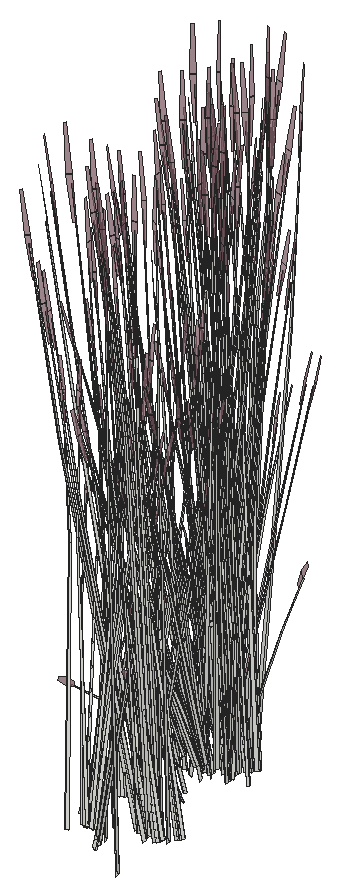
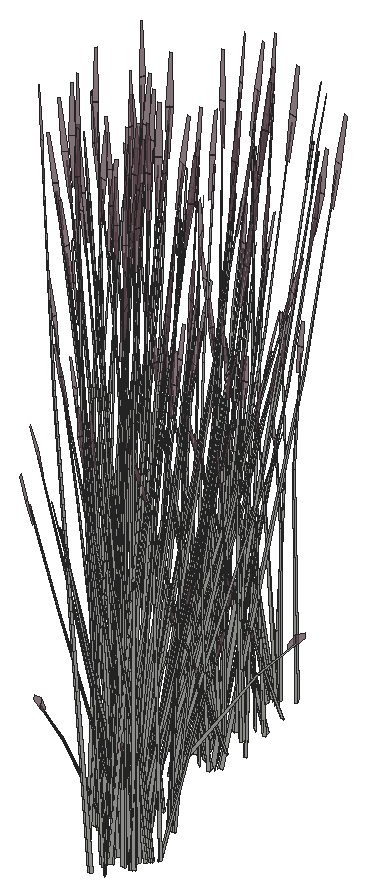
# SketchUp Ruby script. Lengths in inches.
U = 1.inch
M = Sketchup.active_model
def pt(a) = Geom::Point3d.new(a.map { |v| v * U })
def face(e, loops, mat)
  f = e.add_face(loops[0].map { |a| pt(a) })
  loops[1..].each { |l| e.add_face(l.map { |a| pt(a) }).erase! }
  f.material = f.back_material = mat if mat
  f
end
# faces: each face lists its corners as indices into pts; further lists are holes
def faces(e, pts, list, mat = nil) = list.each { |f| face(e, (f[0].is_a?(Array) ? f : [f]).map { |l| l.map { |i| pts[i] } }, mat) }
# xy, xz, yz: faces in a plane at the given z, y or x. An outline is a flat list of corners, or four numbers for a rectangle; further outlines are holes
def ring(l) = l.size == 4 ? [[l[0], l[1]], [l[2], l[1]], [l[2], l[3]], [l[0], l[3]]] : l.each_slice(2).to_a
def flat(e, list, mat, &to3) = list.each { |f| face(e, (f[0].is_a?(Array) ? f : [f]).map { |l| ring(l).map { |u, v| to3.(u, v) } }, mat) }
def xy(e, z, list, mat = nil) = flat(e, list, mat) { |x, y| [x, y, z] }
def xz(e, y, list, mat = nil) = flat(e, list, mat) { |x, z| [x, y, z] }
def yz(e, x, list, mat = nil) = flat(e, list, mat) { |y, z| [x, y, z] }
def lines(e, pts, list) = list.each { |a, b| e.add_line(pt(pts[a]), pt(pts[b])) }
# prism: a flat outline (further loops are holes) pulled along v
def prism(e, loops, v, mat = nil)
  f = face(e, loops, mat); d = Geom::Vector3d.new(v.map { |x| x * U })
  f.pushpull(f.normal.samedirection?(d) ? d.length : -d.length)
end
def box(e, o, s, mat = nil) = prism(e, [[o, [o[0] + s[0], o[1], o[2]], [o[0] + s[0], o[1] + s[1], o[2]], [o[0], o[1] + s[1], o[2]]]], [0, 0, s[2]], mat)
def at(x, y, z, deg = 0) = Geom::Transformation.translation(pt([x, y, z])) * Geom::Transformation.rotation(ORIGIN, Z_AXIS, deg.degrees)
def axes(o, x, y, z) = Geom::Transformation.new([*x, 0, *y, 0, *z, 0, *pt(o).to_a, 1])
def part(name) = M.definitions.add(name)
# library, detail: a bought-in or finely detailed component or shape, given as its bounding box
def library(name, o, s) = part(name).tap { |d| box(d.entities, o, s) }
def detail(e, o, s) = box(e.add_group.entities, o, s)
def put(e, d, t, mat = nil) = e.add_instance(d, t).tap { |i| i.material = mat if mat }
def group(e, t, mat = nil) = e.add_group.tap { |g| g.transformation = t; g.material = mat if mat }.entities
root = M.entities
M.materials.add("LightPink_Translucent").color = [144, 107, 117]
M.materials["LightPink_Translucent"].alpha = 0.75
c1 = part("blade")
p = [[2.15,0.21,22],[0,0.17,0],[0.09,0.45,0],[2.18,0.31,22],[2.29,0.31,22],[0.38,0.45,0],
  [2.48,0.24,33],[2.49,0.24,33],[2.48,0.22,33]]
faces(c1.entities,p,[[0,1,2,3],[4,5,2,3],[6,3,4,7],[8,0,3,6]])
c2 = part("seeds")
p = [[0.3,-0.1,1.38],[-0.01,-0.03,1.59],[-0.01,-0.03,0.03],[0.14,-0.07,-0.07],[0.29,-0.03,3],[0.15,0.01,3.11]]
faces(c2.entities,p,[[0,1,2,3],[1,0,4,5]],"LightPink_Translucent")
c3 = part("blade with seeds")
put(c3.entities,c1,at(0,0,0))
put(c3.entities,c2,axes([2.4,0.25,30.99],[1.5799,-0.05474,1.17369],[-0.12525,1.92788,0.29478],[-0.07173,-0.02425,1.56792]))
put(root,c3,axes([290.63,462.82,5.03],[0.82753,0.35977,-0.1216],[-0.47675,0.52101,-0.67495],[-0.2338,0.18111,1.02557]))
put(root,c3,axes([291.23,468.59,2.48],[0,0.65246,0.49651],[-1.00089,0,0],[0,-0.1486,1.57504]))
put(root,c3,axes([293.6,469.11,2.21],[-0.53742,-0.54764,-0.44739],[0.81403,-0.38564,0.21531],[-0.17391,-0.06776,1.43643]))
put(root,c3,axes([292.09,463.93,5.05],[0.60531,-0.34352,0.35414],[0.573,0.39225,-0.4572],[-0.08718,0.19929,0.87481]))
put(root,c3,axes([293.51,468.92,2.72],[-0.43405,0.58792,0.44739],[-0.90188,-0.28295,-0.21531],[0,-0.13553,1.43643]))
put(root,c3,axes([296.14,462.04,2.84],[-0.02444,-0.61432,1.41272],[1.10603,0.15924,0.59816],[-0.26159,0.33615,1.3335]))
put(root,c3,axes([291.54,464.24,4.73],[-0.73517,-0.0304,0.0643],[0.02016,-0.45906,0.50621],[-0.07693,0.17585,0.77189]))
put(root,c3,axes([291.77,464.28,4.73],[-0.63704,-0.44518,0.48003],[0.67652,-0.38394,0.3958],[-0.11751,0.20886,0.9933]))
put(root,c3,axes([293.8,469.06,2.36],[1.13071,0.13747,0.45755],[-0.23011,0.77639,0.17955],[-0.16524,-0.07497,1.58856]))
put(root,c3,axes([292.125,470.33,2.03],[-0.21015,-0.56852,-0.30978],[0.83462,-0.16144,0.30978],[-0.16826,-0.06556,1.38974]))
put(root,c3,axes([291.77,464.42,4.53],[-0.60531,0.34352,-0.35414],[-0.573,-0.39225,0.4572],[-0.08718,0.19929,0.87481]))
put(root,c3,axes([291.7,464.02,5.4],[0.98321,0.03233,-0.13498],[-0.02687,0.61208,-0.74919],[-0.0683,0.23574,1.13838]))
put(root,c3,axes([293.2,470.3,2.47],[0.96132,-0.17317,0.17642],[0.23737,0.64447,0.35086],[-0.08574,-0.0939,1.60407]))
put(root,c3,axes([292.15,465.75,2.77],[-0.02315,-0.38796,1.1486],[0.57853,0.27671,0.84392],[-0.11378,0.18492,0.25299]))
put(root,c3,axes([291.89,470.57,2.02],[-0.83726,-0.32623,-0.49651],[0.50045,-0.58498,0],[-0.19069,-0.0743,1.57504]))
put(root,c3,axes([294.17,469.42,2.67],[-0.90324,0.43318,-0.29095],[-0.60064,-0.61207,-0.50002],[-0.22285,-0.06216,1.59708]))
put(root,c3,axes([292.37,464.25,5],[0.64041,0.4384,-0.5672],[-0.67652,0.38394,-0.43934],[-0.09744,0.22274,1.08528]))
put(root,c3,axes([291.68,464.91,2.82],[0.8127,-0.11554,0.06507],[0.18684,0.46549,-0.86304],[-0.05152,0.23564,0.7736]))
put(root,c3,axes([294.08,469.61,2.62],[-0.17258,0.58229,0.1448],[-0.84319,-0.10108,-0.41347],[-0.15345,-0.05979,1.26744]))
put(root,c3,axes([292.17,464.05,5.34],[-0.02328,0.60353,-0.7886],[-0.98022,-0.04053,0.09517],[-0.10344,0.25568,1.11556]))
put(root,c3,axes([289.61,465.64,4.71],[0.10149,-0.03939,1.77383],[0.83886,0.26202,-0.16761],[-0.01971,0.21816,0.31391]))
put(root,c3,axes([293.1,463.625,3.875],[-0.0219,-0.25042,1.71376],[0.94901,0.16613,0.13857],[-0.0587,0.35688,0.73262]))
put(root,c3,axes([294.43,470.4,2.2],[-0.90188,-0.29293,0],[0.43405,-0.60866,0],[0,0,1.62707]))
put(root,c3,axes([295.18,469.62,2.46],[-0.87356,-0.52515,-0.25192],[0.73507,-0.5897,0.5513],[-0.23523,0.06143,1.68216]))
put(root,c3,axes([292.88,470.625,2.48],[0.83726,0.32623,0.49651],[-0.50045,0.58498,0],[-0.19069,-0.0743,1.57504]))
put(root,c3,axes([291.48,465.41,2.59],[0.28231,-0.10293,1.43002],[0.69701,0.31035,-0.30754],[-0.20746,0.26854,0.61141]))
put(root,c3,axes([292.4,470.97,2.375],[-0.55932,0.6538,0],[-0.93577,-0.36461,-0.51607],[-0.21313,-0.08304,1.63711]))
put(root,c3,axes([294.74,469.51,2.21],[-0.97146,0.04028,-0.44739],[-0.08785,-0.66859,0.21531],[-0.17391,0.06776,1.43643]))
put(root,c3,axes([291.84,464.9,3.36],[0.01966,-0.33682,1.54345],[0.88405,0.17791,0.21329],[-0.0766,0.35897,0.72882]))
put(root,c3,axes([295.82,471.06,2.19],[-0.55235,-0.65609,-0.05142],[0.93577,-0.36461,0.51607],[-0.23059,0.06247,1.6363]))
put(root,c3,axes([295.5625,470.98,2.03],[-0.83462,-0.16144,-0.30978],[0.21015,-0.56852,0.30978],[-0.16826,0.06556,1.38974]))
put(root,c3,axes([290.94,469.375,5.05],[0.77872,-0.09325,0.35414],[0.20563,0.53305,-0.4572],[-0.22316,0.14318,0.87481]))
put(root,c3,axes([295.42,469.33,2.67],[0.10425,0.7445,-0.29095],[-1.08575,0.04502,-0.50002],[-0.19119,0.09917,1.59708]))
put(root,c3,axes([291.4375,476.32,4.72],[-0.13683,-0.09148,1.74944],[-0.91315,0.058,-0.27667],[-0.14574,-0.2188,0.14031]))
put(root,c3,axes([292.4,477.86,4.98],[-0.42698,-0.53052,-0.71045],[0.87893,-0.29566,0.08574],[-0.09984,-0.25633,1.00501]))
put(root,c3,axes([291.66,476.6875,1.49],[-0.15005,0.02351,1.76342],[-0.82981,-0.26461,-0.26939],[0.01392,-0.22072,0.30037]))
put(root,c3,axes([289.17,470.89,5.65],[0.78943,0.17416,-0.06488],[-0.24284,0.53604,-0.29416],[-0.12912,0.08139,0.97024]))
put(root,c3,axes([294.77,469.9,2.06],[-0.60257,0.49041,-0.62353],[-0.74854,-0.44469,-0.16365],[-0.24146,0.12234,1.37633]))
put(root,c3,axes([295.76,471.23,2.02],[-0.83726,0.32623,-0.49651],[-0.50045,-0.58498,0],[-0.19069,0.0743,1.57504]))
put(root,c3,axes([292.48,477.41,4.53],[0.2697,-0.50175,-0.35414],[0.78684,0.14635,0.4572],[-0.07215,-0.20201,0.87481]))
put(root,c3,axes([290.53,469.33,5.03],[0.82753,0.35977,-0.1216],[-0.47675,0.52101,-0.67495],[-0.2338,0.18111,1.02557]))
put(root,c3,axes([292.07,477.76,4.68],[-0.87941,-0.16356,-0.51099],[0.30143,-0.56078,-0.3958],[-0.08064,-0.22578,0.97773]))
put(root,c3,axes([291.99,470.4375,5.05],[0.60531,-0.34352,0.35414],[0.573,0.39225,-0.4572],[-0.08718,0.19929,0.87481]))
put(root,c3,axes([296.04,468.54,2.84],[-0.02444,-0.61432,1.41272],[1.10603,0.15924,0.59816],[-0.26159,0.33615,1.3335]))
put(root,c3,axes([290.32,477.41,5.09],[0.99656,-0.1677,0.53763],[0.17295,0.65785,0.4433],[-0.23438,-0.19388,1.11249]))
put(root,c3,axes([291.4375,470.75,4.73],[-0.73517,-0.0304,0.0643],[0.02016,-0.45906,0.50621],[-0.07693,0.17585,0.77189]))
put(root,c3,axes([291.67,470.79,4.73],[-0.63704,-0.44518,0.48003],[0.67652,-0.38394,0.3958],[-0.11751,0.20886,0.9933]))
put(root,c3,axes([292.57,477.53,4.73],[0.88151,0.17057,0.48003],[-0.30143,0.56078,0.3958],[-0.05297,-0.22053,0.9933]))
put(root,c3,axes([292.83,477.73,5.03],[-0.87543,0.30377,-0.1216],[-0.4302,-0.53915,-0.67495],[-0.1155,-0.2272,1.02557]))
put(root,c3,axes([292.81,477.49,4.73],[0.6592,-0.22175,0.0643],[0.32265,0.40436,0.50621],[-0.06366,-0.17825,0.77189]))
put(root,c3,axes([290.55,477.55,4.73],[0.4066,-0.41448,0.0643],[0.57901,0.24131,0.50621],[-0.18719,-0.13288,0.77189]))
put(root,c3,axes([290.42,479.86,2.1],[-0.36739,-0.66907,-0.69835],[1.05831,-0.24096,-0.18329],[-0.04061,-0.22656,1.54149]))
put(root,c3,axes([291.67,470.92,4.53],[-0.60531,0.34352,-0.35414],[-0.573,-0.39225,0.4572],[-0.08718,0.19929,0.87481]))
put(root,c3,axes([291.6,470.53,5.4],[0.98321,0.03233,-0.13498],[-0.02687,0.61208,-0.74919],[-0.0683,0.23574,1.13838]))
put(root,c3,axes([292.5625,477.94,5.05],[-0.2697,0.50175,0.35414],[-0.78684,-0.14635,-0.4572],[-0.07215,-0.20201,0.87481]))
put(root,c3,axes([292.06,472.26,2.77],[-0.02315,-0.38796,1.1486],[0.57853,0.27671,0.84392],[-0.11378,0.18492,0.25299]))
put(root,c3,axes([291.5,477.15,2.13],[-0.61821,0.37431,-0.03893],[-0.56645,-0.40995,-0.17649],[-0.03988,-0.11616,0.58215]))
put(root,c3,axes([292.27,470.76,5],[0.64041,0.4384,-0.5672],[-0.67652,0.38394,-0.43934],[-0.09744,0.22274,1.08528]))
put(root,c3,axes([291.58,471.42,2.82],[0.8127,-0.11554,0.06507],[0.18684,0.46549,-0.86304],[-0.05152,0.23564,0.7736]))
put(root,c3,axes([292.07,470.5625,5.34],[-0.02328,0.60353,-0.7886],[-0.98022,-0.04053,0.09517],[-0.10344,0.25568,1.11556]))
put(root,c3,axes([289.51,472.15,4.71],[0.10149,-0.03939,1.77383],[0.83886,0.26202,-0.16761],[-0.01971,0.21816,0.31391]))
put(root,c3,axes([288.25,479.76,2.02],[0,-0.65246,-0.49651],[1.00089,0,0],[0,-0.1486,1.57504]))
put(root,c3,axes([293,470.13,3.875],[-0.0219,-0.25042,1.71376],[0.94901,0.16613,0.13857],[-0.0587,0.35688,0.73262]))
put(root,c3,axes([291.38,471.91,2.59],[0.28231,-0.10293,1.43002],[0.69701,0.31035,-0.30754],[-0.20746,0.26854,0.61141]))
put(root,c3,axes([290.98,480.03,2.21],[0.43405,-0.58792,-0.44739],[0.90188,0.28295,0.21531],[0,-0.13553,1.43643]))
put(root,c3,axes([288.68,479.78,2.03],[0.62448,-0.40708,-0.30978],[0.62448,0.40708,0.30978],[0,-0.13112,1.38974]))
put(root,c3,axes([290.87,480.52,2.67],[-1.00749,-0.31132,-0.29095],[0.48511,-0.65709,-0.50002],[-0.03166,-0.16133,1.59708]))
put(root,c3,axes([291.75,471.41,3.36],[0.01966,-0.33682,1.54345],[0.88405,0.17791,0.21329],[-0.0766,0.35897,0.72882]))
put(root,c3,axes([291.52,480.32,2.43],[1.00799,0.31623,0.24065],[-0.48511,0.65709,0.50002],[0,-0.15147,1.60543]))
put(root,c3,axes([291.125,481.21,2.4375],[0.23711,-0.77313,-0.23429],[1.12425,0.13477,0.51271],[-0.19645,-0.10677,1.5644]))
put(root,c3,axes([291.19,479.88,2.72],[-0.97146,0.04028,0.44739],[-0.08785,-0.66859,-0.21531],[0.17391,-0.06776,1.43643]))
put(root,c3,axes([289.57,483.67,2.59],[-0.25429,0.13207,1.43002],[-0.76157,-0.23115,-0.30754],[0.14117,-0.28747,0.61141]))
put(root,c3,axes([288.68,480.37,2.48],[0,0.65246,0.49651],[-1.00089,0,0],[0,-0.1486,1.57504]))
put(root,c3,axes([291.05,480.9,2.21],[-0.53742,-0.54764,-0.44739],[0.81403,-0.38564,0.21531],[-0.17391,-0.06776,1.43643]))
put(root,c3,axes([291.16,480.12,2.36],[0.38895,0.72959,0.45755],[-1.11135,0.2537,0.17955],[0.01358,-0.13406,1.58856]))
put(root,c3,axes([287.67,482.95,1.49],[-0.15005,0.02351,1.76342],[-0.82981,-0.26461,-0.26939],[0.01392,-0.22072,0.30037]))
put(root,c3,axes([290.96,480.7,2.72],[-0.43405,0.58792,0.44739],[-0.90188,-0.28295,-0.21531],[0,-0.13553,1.43643]))
put(root,c3,axes([292.56,480.18,2.21],[0,-0.75495,0],[1.11865,0,0],[0,0,1.79456]))
put(root,c3,axes([290.1875,484.64,4.98],[0.02328,-0.60353,-0.71045],[0.98022,0.04053,0.08574],[0.10344,-0.25568,1.00501]))
put(root,c3,axes([288.49,483.67,4.53],[0.2697,-0.50175,-0.35414],[0.78684,0.14635,0.4572],[-0.07215,-0.20201,0.87481]))
put(root,c3,axes([291.36,483.23,4.71],[-0.09085,0.04984,1.77383],[-0.89014,-0.16814,-0.16761],[-0.03222,-0.21748,0.31391]))
put(root,c3,axes([292.84,480.77,2.3],[-0.83213,-0.56158,-0.06131],[0.83263,-0.56193,0],[-0.02906,-0.01961,1.75571]))
put(root,c3,axes([290.74,478.73,2.47],[-0.25843,0.64844,0.17642],[-0.9457,-0.1835,0.35086],[0.16336,-0.00316,1.60407]))
put(root,c3,axes([288.63,482.61,2.77],[0.11476,0.38047,1.1486],[-0.63664,-0.21072,0.84392],[0.06851,-0.19481,0.25299]))
put(root,c3,axes([289.99,484.44,4.68],[-0.64041,-0.4384,-0.51099],[0.67652,-0.38394,-0.3958],[0.09744,-0.22274,0.97773]))
put(root,c3,axes([291.26,480.84,2.36],[1.13071,0.13747,0.45755],[-0.23011,0.77639,0.17955],[-0.16524,-0.07497,1.58856]))
put(root,c3,axes([288.59,483.79,4.73],[0.88151,0.17057,0.48003],[-0.30143,0.56078,0.3958],[-0.05297,-0.22053,0.9933]))
put(root,c3,axes([290.66,484.67,5.03],[-0.98321,-0.03233,-0.1216],[0.02687,-0.61208,-0.67495],[0.0683,-0.23574,1.02557]))
put(root,c3,axes([290.59,484.28,4.53],[0.60531,-0.34352,-0.35414],[0.573,0.39225,0.4572],[0.08718,-0.19929,0.87481]))
put(root,c3,axes([290.65,482.08,2.47],[0.96132,-0.17317,0.17642],[0.23737,0.64447,0.35086],[-0.08574,-0.0939,1.60407]))
put(root,c3,axes([288.82,483.75,4.73],[0.6592,-0.22175,0.0643],[0.32265,0.40436,0.50621],[-0.06366,-0.17825,0.77189]))
put(root,c3,axes([292.09,481.93,2.2],[-0.29189,-0.56252,0],[0.83351,-0.19699,0],[0,0,1.54371]))
put(root,c3,axes([291.53,481.39,2.62],[-0.17258,0.58229,0.1448],[-0.84319,-0.10108,-0.41347],[-0.15345,-0.05979,1.26744]))
put(root,c3,axes([293.51,482.11,2.47],[0.25843,-0.64844,0.17642],[0.9457,0.1835,0.35086],[-0.16336,0.00316,1.60407]))
put(root,c3,axes([294.98,480.46,2.47],[-0.70288,-0.47526,0.17642],[0.70832,-0.46097,0.35086],[-0.07763,0.09706,1.60407]))
put(root,c3,axes([290.28,484.77,5.05],[-0.60531,0.34352,0.35414],[-0.573,-0.39225,-0.4572],[0.08718,-0.19929,0.87481]))
put(root,c3,axes([291.89,482.18,2.2],[-0.90188,-0.29293,0],[0.43405,-0.60866,0],[0,0,1.62707]))
put(root,c3,axes([290.33,482.41,2.48],[0.83726,0.32623,0.49651],[-0.50045,0.58498,0],[-0.19069,-0.0743,1.57504]))
put(root,c3,axes([286.29,484.19,2.375],[-0.55932,-0.6538,0],[0.93577,-0.36461,-0.51607],[0.21313,-0.08304,1.63711]))
put(root,c3,axes([293.12,480.49,2.29],[0,0.75458,-0.05637],[-1.11865,0,0],[0,0.02371,1.79368]))
put(root,c3,axes([293.06,480.96,2.72],[0.97146,-0.04028,0.44739],[0.08785,0.66859,-0.21531],[-0.17391,0.06776,1.43643]))
put(root,c3,axes([287.05,484.09,2.02],[0.83726,-0.32623,-0.49651],[0.50045,0.58498,0],[0.19069,-0.0743,1.57504]))
put(root,c3,axes([292.19,481.29,2.21],[-0.97146,0.04028,-0.44739],[-0.08785,-0.66859,0.21531],[-0.17391,0.06776,1.43643]))
put(root,c3,axes([293.27,482.84,2.19],[-0.55235,-0.65609,-0.05142],[0.93577,-0.36461,0.51607],[-0.23059,0.06247,1.6363]))
put(root,c3,axes([293.07,481.25,2.62],[0.66093,0.39201,0.1448],[-0.5513,0.44227,-0.41347],[-0.15345,0.05979,1.26744]))
put(root,c3,axes([286.99,486.29,2.21],[0.43405,-0.58792,-0.44739],[0.90188,0.28295,0.21531],[0,-0.13553,1.43643]))
put(root,c3,axes([287.39,486,2.67],[-0.10425,-0.7445,-0.29095],[1.08575,-0.04502,-0.50002],[0.19119,-0.09917,1.59708]))
put(root,c3,axes([293.77,482.46,2.48],[0.83726,-0.32623,0.49651],[0.50045,0.58498,0],[-0.19069,0.0743,1.57504]))
put(root,c3,axes([287.25,484.35,2.03],[0.83462,0.16144,-0.30978],[-0.21015,0.56852,0.30978],[0.16826,-0.06556,1.38974]))
put(root,c3,axes([292.58,481.95,2.29],[0.38895,0.74956,-0.06012],[-1.11135,0.26265,0],[0.01358,0.02618,1.72173]))
put(root,c3,axes([293.02,482.76,2.03],[-0.83462,-0.16144,-0.30978],[0.21015,-0.56852,0.30978],[-0.16826,0.06556,1.38974]))
put(root,c3,axes([292.87,481.11,2.67],[0.10425,0.7445,-0.29095],[-1.08575,0.04502,-0.50002],[-0.19119,0.09917,1.59708]))
put(root,c3,axes([293.27,480.82,2.21],[-0.43405,0.58792,-0.44739],[-0.90188,-0.28295,0.21531],[0,0.13553,1.43643]))
put(root,c3,axes([287.53,486.58,2.43],[1.00799,0.31623,0.24065],[-0.48511,0.65709,0.50002],[0,-0.15147,1.60543]))
put(root,c3,axes([293.29,482.5,2.33],[1.11998,0.21207,0.30756],[-0.2802,0.75803,-0.36492],[-0.18537,0.09487,1.64885]))
put(root,c3,axes([293.21,483.01,2.02],[-0.83726,0.32623,-0.49651],[-0.50045,-0.58498,0],[-0.19069,0.0743,1.57504]))
put(root,c3,axes([287.21,486.14,2.72],[-0.97146,0.04028,0.44739],[-0.08785,-0.66859,-0.21531],[0.17391,-0.06776,1.43643]))
put(root,c3,axes([287.17,486.38,2.36],[0.38895,0.72959,0.45755],[-1.11135,0.2537,0.17955],[0.01358,-0.13406,1.58856]))
put(root,c3,axes([288.57,486.44,2.21],[0,-0.75495,0],[1.11865,0,0],[0,0,1.79456]))
put(root,c3,axes([289.4375,482.22,5.05],[0.60531,-0.34352,0.35414],[0.573,0.39225,-0.4572],[-0.08718,0.19929,0.87481]))
put(root,c3,axes([293.97,482.91,2.375],[0.55932,0.6538,0],[-0.93577,0.36461,-0.51607],[-0.21313,0.08304,1.63711]))
put(root,c3,axes([289.93,484.7,2.48],[-0.83726,-0.32623,0.49651],[0.50045,-0.58498,0],[0.19069,0.0743,1.57504]))
put(root,c3,axes([293.5,480.32,2.84],[-0.02444,-0.61432,1.41272],[1.10603,0.15924,0.59816],[-0.26159,0.33615,1.3335]))
put(root,c3,axes([288.04,485.97,2.36],[-0.74176,0.59212,0.45755],[-0.88124,-0.52269,0.17955],[0.17882,-0.05909,1.58856]))
put(root,c3,axes([291.14,482.78,5.05],[0.2697,-0.50175,0.35414],[0.78684,0.14635,-0.4572],[0.07215,0.20201,0.87481]))
put(root,c3,axes([288.85,487.03,2.3],[-0.83213,-0.56158,-0.06131],[0.83263,-0.56193,0],[-0.02906,-0.01961,1.75571]))
put(root,c3,axes([286.75,484.99,2.47],[-0.25843,0.64844,0.17642],[-0.9457,-0.1835,0.35086],[0.16336,-0.00316,1.60407]))
put(root,c3,axes([288.73,485.71,2.62],[0.17258,-0.58229,0.1448],[0.84319,0.10108,-0.41347],[0.15345,0.05979,1.26744]))
put(root,c3,axes([288.37,485.87,2.72],[-0.53742,-0.54764,0.44739],[0.81403,-0.38564,-0.21531],[0.17391,0.06776,1.43643]))
put(root,c3,axes([290.89,483.24,4.73],[-0.6592,0.22175,0.0643],[-0.32265,-0.40436,0.50621],[0.06366,0.17825,0.77189]))
put(root,c3,axes([289.05,482.3125,5.4],[0.98321,0.03233,-0.13498],[-0.02687,0.61208,-0.74919],[-0.0683,0.23574,1.13838]))
put(root,c3,axes([289.33,486.61,2.21],[1.00089,0,0],[0,0.67548,0],[0,0,1.78407]))
put(root,c3,axes([291.125,483.19,5.0625],[-0.88151,-0.17057,0.53283],[0.30143,-0.56078,0.43934],[0.05297,0.22053,1.10256]))
put(root,c3,axes([289.61,485.03,2.47],[-0.96132,0.17317,0.17642],[-0.23737,-0.64447,0.35086],[0.08574,0.0939,1.60407]))
put(root,c3,axes([289.51,484.04,2.77],[-0.02315,-0.38796,1.1486],[0.57853,0.27671,0.84392],[-0.11378,0.18492,0.25299]))
put(root,c3,axes([291.03,483.11,1.49],[0.14478,-0.0355,1.76342],[0.8709,0.19542,-0.26939],[0.02547,0.22025,0.30037]))
put(root,c3,axes([289.01,486.27,2.38],[-1.13071,-0.13747,0.49198],[0.23011,-0.77639,0.19306],[0.16524,0.07497,1.70813]))
put(root,c3,axes([289.72,482.54,5],[0.64041,0.4384,-0.5672],[-0.67652,0.38394,-0.43934],[-0.09744,0.22274,1.08528]))
put(root,c3,axes([288.11,488.1875,2.2],[-0.29189,-0.56252,0],[0.83351,-0.19699,0],[0,0,1.54371]))
put(root,c3,axes([289.03,483.2,2.82],[0.8127,-0.11554,0.06507],[0.18684,0.46549,-0.86304],[-0.05152,0.23564,0.7736]))
put(root,c3,axes([289.2,488.11,2.18],[0.93921,-0.22138,-0.19198],[0.33003,0.6377,0.00008],[0.10367,-0.02447,1.73897]))
put(root,c3,axes([289.31,486.9,2.21],[0.62448,0.42144,0],[-0.62448,0.42144,0],[0,0,1.69266]))
put(root,c3,axes([291.22,483.3125,4.53],[-0.2697,0.50175,-0.35414],[-0.78684,-0.14635,0.4572],[0.07215,0.20201,0.87481]))
put(root,c3,axes([291,486.72,2.47],[-0.70288,-0.47526,0.17642],[0.70832,-0.46097,0.35086],[-0.07763,0.09706,1.60407]))
put(root,c3,axes([289.53,482.34,5.34],[-0.02328,0.60353,-0.7886],[-0.98022,-0.04053,0.09517],[-0.10344,0.25568,1.11556]))
